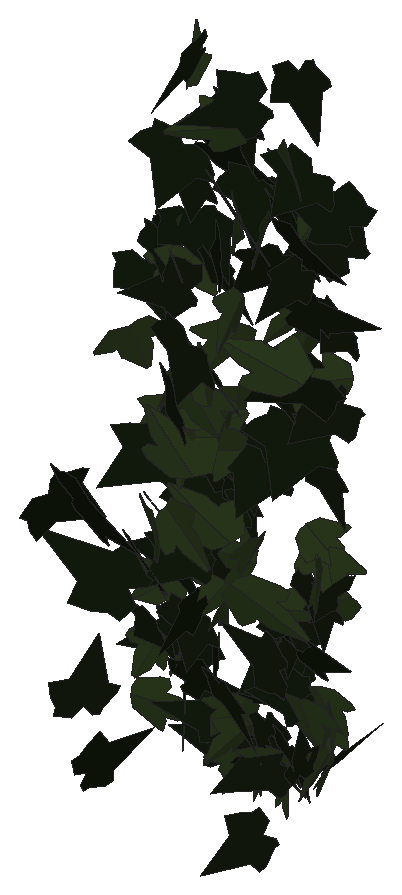
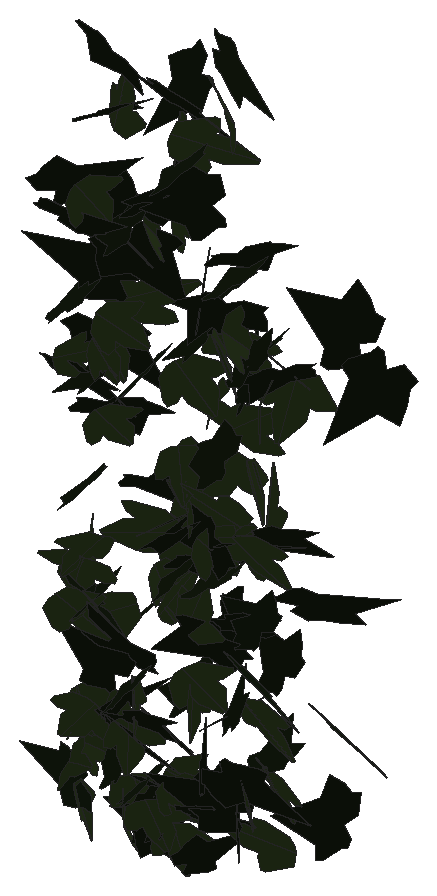
# SketchUp Ruby script. Lengths in inches.
U = 1.inch
M = Sketchup.active_model
def pt(a) = Geom::Point3d.new(a.map { |v| v * U })
def face(e, loops, mat)
  f = e.add_face(loops[0].map { |a| pt(a) })
  loops[1..].each { |l| e.add_face(l.map { |a| pt(a) }).erase! }
  f.material = f.back_material = mat if mat
  f
end
# faces: each face lists its corners as indices into pts; further lists are holes
def faces(e, pts, list, mat = nil) = list.each { |f| face(e, (f[0].is_a?(Array) ? f : [f]).map { |l| l.map { |i| pts[i] } }, mat) }
# xy, xz, yz: faces in a plane at the given z, y or x. An outline is a flat list of corners, or four numbers for a rectangle; further outlines are holes
def ring(l) = l.size == 4 ? [[l[0], l[1]], [l[2], l[1]], [l[2], l[3]], [l[0], l[3]]] : l.each_slice(2).to_a
def flat(e, list, mat, &to3) = list.each { |f| face(e, (f[0].is_a?(Array) ? f : [f]).map { |l| ring(l).map { |u, v| to3.(u, v) } }, mat) }
def xy(e, z, list, mat = nil) = flat(e, list, mat) { |x, y| [x, y, z] }
def xz(e, y, list, mat = nil) = flat(e, list, mat) { |x, z| [x, y, z] }
def yz(e, x, list, mat = nil) = flat(e, list, mat) { |y, z| [x, y, z] }
def lines(e, pts, list) = list.each { |a, b| e.add_line(pt(pts[a]), pt(pts[b])) }
# prism: a flat outline (further loops are holes) pulled along v
def prism(e, loops, v, mat = nil)
  f = face(e, loops, mat); d = Geom::Vector3d.new(v.map { |x| x * U })
  f.pushpull(f.normal.samedirection?(d) ? d.length : -d.length)
end
def box(e, o, s, mat = nil) = prism(e, [[o, [o[0] + s[0], o[1], o[2]], [o[0] + s[0], o[1] + s[1], o[2]], [o[0], o[1] + s[1], o[2]]]], [0, 0, s[2]], mat)
def at(x, y, z, deg = 0) = Geom::Transformation.translation(pt([x, y, z])) * Geom::Transformation.rotation(ORIGIN, Z_AXIS, deg.degrees)
def axes(o, x, y, z) = Geom::Transformation.new([*x, 0, *y, 0, *z, 0, *pt(o).to_a, 1])
def part(name) = M.definitions.add(name)
# library, detail: a bought-in or finely detailed component or shape, given as its bounding box
def library(name, o, s) = part(name).tap { |d| box(d.entities, o, s) }
def detail(e, o, s) = box(e.add_group.entities, o, s)
def put(e, d, t, mat = nil) = e.add_instance(d, t).tap { |i| i.material = mat if mat }
def group(e, t, mat = nil) = e.add_group.tap { |g| g.transformation = t; g.material = mat if mat }.entities
root = M.entities
M.materials.add("1026 AP 7946 SUNNY SIDE UP").color = [254, 231, 186]
M.materials.add("efeu1").color = [18, 25, 13]
M.materials.add("efeu2").color = [43, 57, 29]
c1 = part("ivyleaf_9")
p = [[1.54,2.16,1.25],[1.36,2.04,1.19],[-0.21,0.99,0.68],[-0.71,1.11,0.82],[-0.85,0.86,0.67],[-0.8,0.17,0.21],
  [-0.9,-0.01,0.1],[-0.67,-0.16,-0.02],[-0.08,-0.08,-0.05],[-0.03,-0.6,-0.4],[0.65,-0.88,-0.66],[0.83,-0.6,-0.49],
  [1.29,-0.42,-0.43],[1.8125,-0.07,-0.26],[1.21,0.44,0.15]]
faces(c1.entities,p,[[0,1,2,3,4,5,6,7,8,9,10,11,12,13,14]],"efeu1")
c2 = part("ivyleaf_10")
p = [[0,0.5,-0.03],[-0.0625,2.02,-0.43],[-0.19,2.01,-0.46],[-0.54,1.05,-0.29],[-0.52,0.625,-0.18],[-0.83,0.76,-0.28],
  [-1.16,0.64,-0.33],[-1.15,0.33,-0.24],[-0.77,-0.39,0.02],[-0.3,-0.51,0.16],[0.04,-0.48,0.23],[-0.02,2.01,-0.4375],
  [-0.06,2.01,-0.43],[0.04,-0.49,0.23],[0.67,-0.49,0.14],[1.38,0.36,-0.2],[1.375,0.51,-0.24],[0.81,0.65,-0.19],
  [0.62,0.59,-0.15],[0.6,1.09,-0.28],[0.5,1.23,-0.31]]
faces(c2.entities,p,[[0,1,2,3,4,5,6,7,8,9,10],[11,12,0,13,14,15,16,17,18,19,20]],"efeu2")
put(root,c1,axes([114.62,207.98,273.75],[0.2482,-0.1981,0.34373],[0.28085,-0.28405,-0.26157],[0.54338,0.2373,-0.02181]),"1026 AP 7946 SUNNY SIDE UP")
put(root,c1,axes([114.02,208.15,273.55],[-0.02229,-0.02198,-0.42734],[-0.23875,0.38648,-0.01349],[0.60777,0.15101,-0.02098]),"1026 AP 7946 SUNNY SIDE UP")
put(root,c1,axes([116.61,209.73,268.14],[-0.49831,0.10185,-0.0594],[0.071,-0.04894,-0.3416],[-0.17027,-0.31848,0.0314]),"1026 AP 7946 SUNNY SIDE UP")
put(root,c1,axes([114.91,210.2,275.41],[-0.06712,-0.30626,0.23486],[-0.02015,-0.22987,-0.31951],[0.60163,-0.04187,0.0155]),"1026 AP 7946 SUNNY SIDE UP")
put(root,c1,axes([115.61,210.05,278.29],[0.50276,-0.19479,-0.12293],[-0.18455,0.0338,-0.38421],[0.30709,0.33922,-0.02965]),"1026 AP 7946 SUNNY SIDE UP")
put(root,c2,axes([114.29,210.19,272.0625],[-0.33314,0.25497,0.19565],[0.21856,-0.12904,0.34006],[0.44809,0.2525,-0.02041]),"1026 AP 7946 SUNNY SIDE UP")
put(root,c1,axes([113.23,209.89,269.08],[-0.44459,0.21006,-0.05411],[-0.04291,0.05309,0.36219],[0.33822,0.28286,-0.02517]),"1026 AP 7946 SUNNY SIDE UP")
put(root,c2,axes([115.65,210.34,276.28],[-0.00744,-0.21724,0.27933],[0.17282,-0.25942,-0.2127],[0.51985,0.08313,0.07471]),"1026 AP 7946 SUNNY SIDE UP")
put(root,c1,axes([113.74,210.18,271.05],[-0.41644,-0.23212,-0.14016],[-0.18031,-0.07327,0.36183],[-0.38155,0.28797,-0.01802]),"1026 AP 7946 SUNNY SIDE UP")
put(root,c1,axes([114.44,210.51,274.11],[-0.06511,-0.04806,0.37115],[-0.04374,-0.36139,-0.05504],[0.57026,-0.03321,0.03815]),"1026 AP 7946 SUNNY SIDE UP")
put(root,c1,axes([113.22,210.04,267.89],[0.04851,0.05898,0.37667],[0.39457,0.26605,-0.06453],[-0.42758,0.2522,-0.01681]),"1026 AP 7946 SUNNY SIDE UP")
put(root,c2,axes([114.75,210.3,273.41],[0.47491,0.06702,0.23386],[-0.35843,-0.01444,0.31728],[0.09807,-0.37732,0.02712]),"1026 AP 7946 SUNNY SIDE UP")
put(root,c2,axes([115.82,210.4375,271.53],[-0.30148,0.00089,-0.33899],[0.50697,-0.07563,-0.19419],[-0.10344,-0.37326,0.03626]),"1026 AP 7946 SUNNY SIDE UP")
put(root,c1,axes([114.61,210.74,270.83],[-0.11614,0.01292,-0.32557],[0.28583,-0.26394,-0.05641],[-0.40715,-0.18898,0.05327]),"1026 AP 7946 SUNNY SIDE UP")
put(root,c2,axes([115.58,210.43,277.7],[0.19843,-0.25846,-0.2104],[0.03101,0.22278,-0.2786],[0.51561,0.08607,0.09772]),"1026 AP 7946 SUNNY SIDE UP")
put(root,c1,axes([116.1,210.73,270.28],[-0.02052,-0.33182,0.01504],[0.00434,0.01639,0.34219],[-0.52238,0.01317,0.00225]),"1026 AP 7946 SUNNY SIDE UP")
put(root,c1,axes([115.0625,210.77,269.59],[0.21253,-0.27319,0.10023],[0.05342,-0.09341,-0.31437],[0.45369,0.13897,-0.00994]),"1026 AP 7946 SUNNY SIDE UP")
put(root,c2,axes([114.13,210.79,272.02],[0.23931,-0.02385,0.34986],[0.51535,-0.09094,-0.15836],[0.14563,0.361,-0.01452]),"1026 AP 7946 SUNNY SIDE UP")
put(root,c2,axes([116.14,210.875,275.09],[0.19966,0.1981,0.32347],[-0.33152,-0.23322,0.23892],[0.47868,-0.24416,0.03055]),"1026 AP 7946 SUNNY SIDE UP")
put(root,c2,axes([114.28,210.89,273.34],[0.33771,-0.16744,0.17796],[0.18613,-0.1295,-0.28015],[0.33056,0.24398,-0.02407]),"1026 AP 7946 SUNNY SIDE UP")
put(root,c2,axes([114.94,210.86,272.1],[0.32041,0.10412,0.28335],[-0.43817,-0.03639,0.22715],[0.14506,-0.33989,0.06028]),"1026 AP 7946 SUNNY SIDE UP")
put(root,c2,axes([113.32,210.88,274.8],[-0.26462,-0.30768,-0.14131],[0.11753,0.1134,-0.36046],[0.51535,-0.18385,0.00965]),"1026 AP 7946 SUNNY SIDE UP")
put(root,c2,axes([114.85,211.29,273.19],[-0.04701,-0.07544,-0.32505],[-0.29559,-0.25369,0.07946],[-0.41494,0.18927,-0.01978]),"1026 AP 7946 SUNNY SIDE UP")
put(root,c1,axes([114.26,211.21,279.59],[-0.37275,0.17604,-0.228],[0.2485,-0.15858,-0.30389],[-0.37022,-0.28368,0.02558]),"1026 AP 7946 SUNNY SIDE UP")
put(root,c1,axes([113.14,211.35,270.75],[0.06292,-0.16076,0.29588],[0.14529,-0.27316,-0.17184],[0.49803,0.1,0.01275]),"1026 AP 7946 SUNNY SIDE UP")
put(root,c1,axes([116.38,210.9375,268.58],[0.06624,0.0945,0.26304],[-0.05065,0.25775,-0.09149],[-0.42429,-0.01602,0.05199]),"1026 AP 7946 SUNNY SIDE UP")
put(root,c2,axes([114.92,211.35,268.58],[-0.06145,-0.18285,0.24697],[-0.02077,-0.24151,-0.19257],[0.47494,-0.03422,0.02354]),"1026 AP 7946 SUNNY SIDE UP")
put(root,c2,axes([114.54,211,274.17],[-0.04366,0.27735,-0.1678],[-0.04019,0.16266,0.28799],[0.50542,0.03689,0.0084]),"1026 AP 7946 SUNNY SIDE UP")
put(root,c1,axes([113.53,211.37,272.68],[-0.41707,-0.16252,0.1354],[-0.15216,-0.0944,-0.31976],[0.29235,-0.28099,0.02674]),"1026 AP 7946 SUNNY SIDE UP")
put(root,c2,axes([116.4,211.38,268.5625],[0.07382,-0.16814,0.26457],[0.11941,-0.24636,-0.18124],[0.46896,0.0892,0.0045]),"1026 AP 7946 SUNNY SIDE UP")
put(root,c1,axes([116.17,211.43,278.16],[-0.28513,-0.22686,0.14425],[-0.04325,-0.15402,-0.29199],[0.41803,-0.17067,0.06818]),"1026 AP 7946 SUNNY SIDE UP")
put(root,c1,axes([114.06,211.35,271.23],[-0.36398,-0.14775,0.07439],[-0.0783,-0.05738,-0.28243],[0.24706,-0.23586,0.0201]),"1026 AP 7946 SUNNY SIDE UP")
put(root,c2,axes([116,211.21,278.06],[-0.41765,0.22798,0.02135],[0.0447,0.00333,0.35998],[0.357,0.2663,-0.02009]),"1026 AP 7946 SUNNY SIDE UP")
put(root,c1,axes([116.02,211.41,273.83],[-0.37975,-0.25076,-0.02997],[0.05641,0.00378,-0.35785],[0.39266,-0.24306,0.02243]),"1026 AP 7946 SUNNY SIDE UP")
put(root,c1,axes([115.6,211.36,268.26],[-0.48011,-0.00343,0.03807],[-0.05734,-0.02996,-0.31329],[0.01098,-0.3061,0.02843]),"1026 AP 7946 SUNNY SIDE UP")
put(root,c1,axes([116.24,211.31,274.88],[0.11343,0.02058,-0.34173],[-0.39286,-0.22066,-0.07134],[-0.34489,0.25812,-0.03112]),"1026 AP 7946 SUNNY SIDE UP")
put(root,c2,axes([116.26,211.48,271.52],[0.07278,-0.04443,0.33542],[0.3182,-0.25553,-0.067],[0.40761,0.20742,-0.00759]),"1026 AP 7946 SUNNY SIDE UP")
put(root,c1,axes([114.05,211.24,275.6],[-0.39008,0.18656,0.09253],[-0.14389,0.02513,-0.31775],[-0.29125,-0.26228,0.03305]),"1026 AP 7946 SUNNY SIDE UP")
put(root,c1,axes([115.75,211.48,268.51],[0.12541,-0.23672,0.15952],[0.04616,-0.15448,-0.25756],[0.44355,0.08301,-0.01829]),"1026 AP 7946 SUNNY SIDE UP")
put(root,c1,axes([115.96,211.42,276.47],[-0.45666,0.04908,-0.12472],[0.1783,-0.05318,-0.30206],[-0.10281,-0.31023,0.03014]),"1026 AP 7946 SUNNY SIDE UP")
put(root,c1,axes([115.25,211.5,273.01],[-0.3177,-0.20742,-0.00521],[0.02705,-0.01136,-0.29764],[0.32507,-0.20176,0.01968]),"1026 AP 7946 SUNNY SIDE UP")
put(root,c1,axes([114.31,211.53,272.17],[-0.26387,-0.29403,-0.02556],[0.04593,0.00992,-0.34808],[0.46148,-0.16911,0.02003]),"1026 AP 7946 SUNNY SIDE UP")
put(root,c2,axes([114.57,211.54,278.33],[-0.10653,-0.03707,0.34364],[-0.33223,-0.25997,-0.07544],[0.41046,-0.22004,0.02812]),"1026 AP 7946 SUNNY SIDE UP")
put(root,c1,axes([115.76,211.52,276.81],[0.17683,-0.14292,0.29286],[0.2571,-0.23369,-0.18851],[0.43052,0.19826,-0.00771]),"1026 AP 7946 SUNNY SIDE UP")
put(root,c2,axes([115.09,211.56,267.95],[-0.06022,0.08972,-0.28633],[0.07867,-0.27468,-0.09987],[-0.45322,-0.0596,0.02071]),"1026 AP 7946 SUNNY SIDE UP")
put(root,c1,axes([115.86,211.57,269.33],[-0.14624,-0.02373,0.27968],[-0.27618,-0.21428,-0.08249],[0.3279,-0.19106,0.05525]),"1026 AP 7946 SUNNY SIDE UP")
put(root,c2,axes([116.1,211.375,269.36],[-0.4555,0.03515,-0.04957],[0.06964,-0.03423,-0.2994],[-0.06306,-0.29168,0.02741]),"1026 AP 7946 SUNNY SIDE UP")
put(root,c2,axes([114.86,211.58,271.25],[-0.04933,0.19465,0.27143],[0.08984,-0.25624,0.20138],[0.50577,0.0645,-0.0093]),"1026 AP 7946 SUNNY SIDE UP")
put(root,c1,axes([113.87,211.6,269.97],[-0.09179,-0.27319,0.09744],[0.00866,-0.0991,-0.28725],[0.45531,-0.05319,0.02511]),"1026 AP 7946 SUNNY SIDE UP")
put(root,c1,axes([113.18,211.63,269.51],[-0.21964,-0.09653,0.24476],[0.02359,-0.27365,-0.10681],[0.40335,-0.03656,0.13953]),"1026 AP 7946 SUNNY SIDE UP")
put(root,c1,axes([113.35,211.6,271.43],[0.11701,-0.19171,0.2225],[0.17016,-0.18948,-0.21172],[0.42239,0.12944,0.02366]),"1026 AP 7946 SUNNY SIDE UP")
put(root,c1,axes([115.07,211.51,278.92],[-0.5162,0.09639,0.0505],[-0.08921,-0.02219,-0.35055],[-0.14429,-0.3311,0.03608]),"1026 AP 7946 SUNNY SIDE UP")
put(root,c2,axes([115.5,211.49,268.29],[-0.32768,-0.17493,0.08808],[-0.08486,-0.06994,-0.2801],[0.29489,-0.21451,0.01727]),"1026 AP 7946 SUNNY SIDE UP")
put(root,c2,axes([115.15,211.63,276.87],[0.18633,-0.17931,0.23549],[0.18012,-0.19923,-0.22236],[0.42119,0.16452,-0.00909]),"1026 AP 7946 SUNNY SIDE UP")
put(root,c1,axes([115.875,211.45,275.78],[0.18203,-0.00969,0.3262],[0.45421,-0.1353,-0.11384],[0.20469,0.30885,-0.03748]),"1026 AP 7946 SUNNY SIDE UP")
put(root,c1,axes([115.54,211.54,276.51],[0.06927,0.17335,-0.28918],[-0.12559,-0.27019,-0.18574],[-0.50468,0.09103,0.00653]),"1026 AP 7946 SUNNY SIDE UP")
put(root,c2,axes([115.04,211.54,271.62],[0.00025,-0.29987,0.04476],[0.00009,-0.04515,-0.30919],[0.47683,0.00017,0.00003]),"1026 AP 7946 SUNNY SIDE UP")
put(root,c2,axes([115.5,211.6875,267.8],[0.12953,-0.05535,0.29042],[0.30217,-0.20783,-0.10099],[0.33646,0.20796,-0.02111]),"1026 AP 7946 SUNNY SIDE UP")
put(root,c2,axes([114.57,211.65,274.89],[-0.23102,-0.26351,0.17505],[-0.05216,-0.17516,-0.30771],[0.49153,-0.14244,0.04962]),"1026 AP 7946 SUNNY SIDE UP")
put(root,c1,axes([115.22,211.55,274.71],[0.22419,-0.283,-0.09671],[-0.0821,0.07694,-0.32579],[0.46079,0.1514,-0.011]),"1026 AP 7946 SUNNY SIDE UP")
put(root,c2,axes([113.98,211.51,273.71],[-0.48706,-0.06532,-0.13138],[0.20862,-0.01839,-0.32333],[0.08368,-0.33433,0.04142]),"1026 AP 7946 SUNNY SIDE UP")
put(root,c1,axes([114.24,211.76,275.89],[-0.02599,0.04091,0.33293],[-0.09965,-0.31757,0.03625],[0.50206,-0.06092,0.02443]),"1026 AP 7946 SUNNY SIDE UP")
put(root,c2,axes([116.34,211.6875,269.23],[-0.06933,0.17317,-0.20936],[0.06867,-0.19953,-0.1852],[-0.41537,-0.06189,0.00433]),"1026 AP 7946 SUNNY SIDE UP")
put(root,c2,axes([113.12,211.62,269.32],[0.40185,-0.18584,-0.02249],[-0.04965,-0.00821,-0.32455],[0.28982,0.25628,-0.02442]),"1026 AP 7946 SUNNY SIDE UP")
put(root,c1,axes([116.5,211.7,274.35],[-0.52552,-0.00842,-0.0104],[0.01703,-0.03295,-0.34291],[0.01162,-0.33274,0.03225]),"1026 AP 7946 SUNNY SIDE UP")
put(root,c2,axes([113.48,211.57,273.72],[0.12337,-0.28271,-0.08316],[-0.03456,0.076,-0.30181],[0.46032,0.08148,-0.00037]),"1026 AP 7946 SUNNY SIDE UP")
put(root,c1,axes([113.58,211.77,268.53],[-0.05298,-0.01654,-0.30284],[0.40257,-0.14758,-0.02255],[-0.22834,-0.25636,0.03051]),"1026 AP 7946 SUNNY SIDE UP")
put(root,c1,axes([112.97,211.65,275.47],[-0.0378,-0.28014,-0.13285],[0.05584,0.12437,-0.288],[0.48065,-0.03648,0.02301]),"1026 AP 7946 SUNNY SIDE UP")
put(root,c1,axes([115.99,211.83,271.06],[0.0335,-0.29784,0.15273],[0.0072,-0.14998,-0.30844],[0.52428,0.02109,-0.00552]),"1026 AP 7946 SUNNY SIDE UP")
put(root,c2,axes([115.74,211.43,270.85],[-0.04182,-0.06601,-0.29638],[0.30756,0.21189,-0.06756],[0.34683,-0.19586,0.02418]),"1026 AP 7946 SUNNY SIDE UP")
put(root,c1,axes([115.73,211.73,270.04],[0.10462,-0.08213,0.29047],[0.28629,-0.21591,-0.11013],[0.36322,0.19384,0.00314]),"1026 AP 7946 SUNNY SIDE UP")
put(root,c2,axes([113,211.64,268.32],[0.01434,-0.02948,-0.32352],[0.48721,-0.05705,0.01446],[-0.09138,-0.30878,0.02633]),"1026 AP 7946 SUNNY SIDE UP")
put(root,c2,axes([114.68,211.68,267.92],[-0.27109,-0.19139,0.0564],[-0.03384,-0.05552,-0.26483],[0.31165,-0.17251,0.02031]),"1026 AP 7946 SUNNY SIDE UP")
put(root,c2,axes([113.66,211.71,275.7],[0.4504,0.05989,-0.14816],[-0.21241,-0.05588,-0.30076],[-0.12302,0.31576,-0.02315]),"1026 AP 7946 SUNNY SIDE UP")
put(root,c1,axes([114.9,211.8,277.4],[-0.16549,-0.29489,-0.01607],[0.01458,0.01147,-0.32245],[0.46397,-0.10554,0.0044]),"1026 AP 7946 SUNNY SIDE UP")
put(root,c1,axes([114.34,211.72,268.36],[-0.25704,0.06606,0.20435],[-0.32788,-0.04079,-0.16359],[-0.01423,-0.25349,0.07795]),"1026 AP 7946 SUNNY SIDE UP")
put(root,c2,axes([114.58,211.77,268.69],[-0.21309,-0.19735,0.15338],[-0.08056,-0.14497,-0.24502],[0.38137,-0.1409,0.03395]),"1026 AP 7946 SUNNY SIDE UP")
put(root,c1,axes([114.89,211.79,268.15],[0.24192,-0.19898,0.18962],[0.16936,-0.15076,-0.25993],[0.39243,0.18772,-0.00472]),"1026 AP 7946 SUNNY SIDE UP")
put(root,c1,axes([116.51,211.57,271.24],[-0.26812,0.25713,0.06017],[-0.08185,0.0336,-0.31665],[-0.40594,-0.17661,0.02411]),"1026 AP 7946 SUNNY SIDE UP")
put(root,c1,axes([114.99,211.74,268.03],[-0.06458,0.15674,-0.21547],[0.06648,-0.20586,-0.16798],[-0.40669,-0.05854,0.00676]),"1026 AP 7946 SUNNY SIDE UP")
put(root,c1,axes([115.14,211.73,268.59],[0.18615,-0.26162,-0.0448],[-0.02637,0.03852,-0.2956],[0.4158,0.11957,0.00131]),"1026 AP 7946 SUNNY SIDE UP")
put(root,c2,axes([116.33,211.9,274.63],[-0.06983,0.04405,0.30587],[-0.05695,-0.29848,0.03832],[0.46812,-0.02974,0.05029]),"1026 AP 7946 SUNNY SIDE UP")
put(root,c1,axes([113.13,211.89,275.76],[0.01647,-0.28515,0.11083],[0.00017,-0.10926,-0.29457],[0.48012,0.00982,-0.0037]),"1026 AP 7946 SUNNY SIDE UP")
put(root,c1,axes([115.64,211.84,279.44],[-0.21032,-0.1066,-0.29479],[0.47384,0.00052,-0.14562],[0.07188,-0.31532,0.09736]),"1026 AP 7946 SUNNY SIDE UP")
put(root,c1,axes([113.65,211.9,272.7],[-0.33419,-0.02522,0.19326],[-0.23595,-0.14979,-0.19661],[0.18178,-0.24079,0.1001]),"1026 AP 7946 SUNNY SIDE UP")
put(root,c2,axes([114.41,211.6875,271.23],[-0.43068,0.15889,-0.07601],[-0.07964,0.061,0.32541],[0.26432,0.27727,-0.0258]),"1026 AP 7946 SUNNY SIDE UP")
put(root,c1,axes([115.62,211.64,270.3125],[-0.33927,0.13586,0.177],[0.23525,-0.08325,0.26207],[0.25026,0.26245,-0.0064]),"1026 AP 7946 SUNNY SIDE UP")
put(root,c1,axes([113.96,211.7,271.14],[-0.00956,-0.08492,-0.28627],[0.32455,0.19371,-0.06462],[0.32056,-0.19865,0.05688]),"1026 AP 7946 SUNNY SIDE UP")
put(root,c2,axes([114.22,211.92,270.54],[-0.23378,-0.19982,0.19993],[-0.05444,-0.20624,-0.24587],[0.43585,-0.13294,0.07652]),"1026 AP 7946 SUNNY SIDE UP")
put(root,c2,axes([115.69,211.85,275.05],[-0.07072,-0.27578,0.09656],[0.01608,-0.09786,-0.28733],[0.45852,-0.03911,0.02497]),"1026 AP 7946 SUNNY SIDE UP")
put(root,c2,axes([113.3,211.75,270.31],[0.36191,-0.1317,-0.18318],[-0.26035,0.06607,-0.27197],[0.22939,0.28277,-0.01966]),"1026 AP 7946 SUNNY SIDE UP")
put(root,c1,axes([114.06,211.9,269.03],[-0.01933,0.10876,0.26695],[-0.0981,-0.25333,0.10526],[0.42994,-0.05291,0.03602]),"1026 AP 7946 SUNNY SIDE UP")
put(root,c1,axes([116.26,212.02,275.44],[-0.13567,-0.17192,0.24799],[-0.01643,-0.2498,-0.18835],[0.46608,-0.05884,0.06555]),"1026 AP 7946 SUNNY SIDE UP")
put(root,c2,axes([113.86,211.61,278.92],[0.31926,-0.18133,0.26626],[-0.2622,0.20077,0.28013],[-0.42311,-0.26125,0.02731]),"1026 AP 7946 SUNNY SIDE UP")
put(root,c2,axes([115.68,211.95,273.95],[-0.2174,-0.17602,0.19137],[-0.01042,-0.20962,-0.20981],[0.40341,-0.10027,0.09771]),"1026 AP 7946 SUNNY SIDE UP")
put(root,c2,axes([115.57,211.98,275.46],[-0.09651,-0.19956,0.24018],[-0.07025,-0.23058,-0.21575],[0.47878,-0.07406,0.01676]),"1026 AP 7946 SUNNY SIDE UP")
put(root,c2,axes([116.09,211.8,269.36],[-0.38423,0.02888,-0.12019],[0.17468,-0.04755,-0.25176],[-0.07277,-0.26664,0.03025]),"1026 AP 7946 SUNNY SIDE UP")
put(root,c2,axes([113.91,211.99,272.67],[-0.06553,-0.23276,0.22396],[0.01644,-0.22145,-0.24202],[0.50195,-0.02313,0.03716]),"1026 AP 7946 SUNNY SIDE UP")
put(root,c2,axes([113.82,211.71,272.99],[0.33062,0.01429,-0.27454],[0.40931,0.06426,0.21545],[0.09306,-0.33338,0.02773]),"1026 AP 7946 SUNNY SIDE UP")
put(root,c1,axes([114.2,211.98,267.82],[-0.07617,0.00683,0.28909],[-0.3549,-0.17018,-0.03687],[0.2623,-0.22827,0.03406]),"1026 AP 7946 SUNNY SIDE UP")
put(root,c1,axes([115.69,211.83,269.34],[-0.37947,0.11767,0.09346],[-0.14007,0.02231,-0.27585],[-0.18619,-0.25662,0.01704]),"1026 AP 7946 SUNNY SIDE UP")
put(root,c1,axes([115.28,211.98,269.63],[-0.36981,-0.12254,0.04337],[-0.04481,-0.03766,-0.27265],[0.19911,-0.23606,0.01919]),"1026 AP 7946 SUNNY SIDE UP")
put(root,c1,axes([113.64,211.83,268.72],[0.21054,-0.03248,0.28533],[0.39571,-0.11876,-0.14028],[0.18958,0.28397,-0.02406]),"1026 AP 7946 SUNNY SIDE UP")
put(root,c1,axes([116.4,211.97,277.17],[-0.04866,0.04832,0.34079],[-0.4998,-0.10632,-0.01527],[0.16149,-0.31448,0.05543]),"1026 AP 7946 SUNNY SIDE UP")
put(root,c1,axes([114.02,211.83,277.7],[0.42745,-0.07822,0.17101],[0.23445,-0.08014,-0.29015],[0.16928,0.30851,-0.02996]),"1026 AP 7946 SUNNY SIDE UP")
put(root,c2,axes([116.3,211.95,270.95],[-0.23347,-0.11718,0.21765],[-0.22923,-0.15526,-0.19456],[0.30407,-0.20702,0.02044]),"1026 AP 7946 SUNNY SIDE UP")
put(root,c1,axes([113.3,212.06,277.33],[-0.26024,-0.28835,0.04591],[-0.01081,-0.04925,-0.34227],[0.45906,-0.16462,0.01797]),"1026 AP 7946 SUNNY SIDE UP")
put(root,c1,axes([113.84,212.07,272.12],[-0.09155,-0.23129,0.15307],[0.0624,-0.15864,-0.23722],[0.42886,-0.02629,0.06719]),"1026 AP 7946 SUNNY SIDE UP")
put(root,c1,axes([113.65,212,274.06],[0.25591,-0.24689,0.13905],[0.09369,-0.1238,-0.30487],[0.43348,0.17251,-0.01619]),"1026 AP 7946 SUNNY SIDE UP")
put(root,c2,axes([113.43,211.86,269.21],[0.1882,-0.25212,-0.05521],[-0.02155,0.0512,-0.28705],[0.40426,0.1201,0.0104]),"1026 AP 7946 SUNNY SIDE UP")
put(root,c1,axes([113.46,211.76,270.85],[-0.24786,0.22081,0.12416],[-0.13923,0.08285,-0.2781],[-0.36924,-0.17946,0.02152]),"1026 AP 7946 SUNNY SIDE UP")
put(root,c1,axes([114.01,211.91,275.8],[0.25772,-0.25706,-0.0366],[-0.03982,0.02424,-0.31381],[0.40579,0.16564,-0.00756]),"1026 AP 7946 SUNNY SIDE UP")
put(root,c2,axes([116.09,211.88,271.6],[0.43199,0.10045,0.07164],[0.11376,0.00241,-0.30048],[-0.15416,0.28325,-0.02098]),"1026 AP 7946 SUNNY SIDE UP")
put(root,c2,axes([115.28,211.79,269.96],[0.11575,-0.2512,-0.14176],[0.00399,0.14119,-0.26608],[0.44927,0.06347,0.03888]),"1026 AP 7946 SUNNY SIDE UP")
put(root,c1,axes([113.44,212.07,270.25],[-0.09284,-0.0287,0.28995],[-0.04442,-0.28564,-0.03776],[0.44288,-0.03467,0.05699]),"1026 AP 7946 SUNNY SIDE UP")
put(root,c1,axes([114.4,212.03,272.03],[0.10543,-0.26447,0.07585],[0.00333,-0.07684,-0.28103],[0.4323,0.06509,-0.01633]),"1026 AP 7946 SUNNY SIDE UP")
put(root,c1,axes([113.1,212.12,275.68],[0.02833,-0.20987,0.25527],[0.06398,-0.24596,-0.21805],[0.50801,0.04268,0.01322]),"1026 AP 7946 SUNNY SIDE UP")
put(root,c2,axes([114.44,211.89,273.76],[-0.21898,-0.26539,-0.01082],[0.01812,0.00411,-0.30862],[0.41715,-0.1395,0.00773]),"1026 AP 7946 SUNNY SIDE UP")
put(root,c1,axes([115.74,211.92,274.6875],[0.26728,-0.23501,-0.04753],[-0.01495,0.04829,-0.29778],[0.37589,0.16903,0.02196]),"1026 AP 7946 SUNNY SIDE UP")
put(root,c1,axes([113.82,211.99,272.84],[-0.02956,-0.04991,-0.3273],[0.50198,0.03323,-0.02466],[0.05741,-0.31624,0.04715]),"1026 AP 7946 SUNNY SIDE UP")
put(root,c1,axes([115.2,212.02,277.02],[0.22446,-0.26932,0.07575],[0.04024,-0.07134,-0.31424],[0.43777,0.14465,-0.00995]),"1026 AP 7946 SUNNY SIDE UP")
put(root,c2,axes([114.26,211.82,270.23],[0.04048,-0.25039,-0.14764],[0.01584,0.14315,-0.25752],[0.45226,0.0174,0.02223]),"1026 AP 7946 SUNNY SIDE UP")
put(root,c1,axes([113.68,211.91,276.34],[-0.15779,-0.21161,-0.23146],[0.16119,0.19865,-0.24004],[0.4563,-0.14335,0.00476]),"1026 AP 7946 SUNNY SIDE UP")
put(root,c2,axes([116.09,211.93,268.14],[0.11059,-0.26758,-0.02727],[-0.01281,0.02366,-0.28488],[0.42238,0.07078,-0.0015]),"1026 AP 7946 SUNNY SIDE UP")
put(root,c1,axes([115.18,212.125,270.08],[0.01841,-0.26326,0.14825],[-0.01082,-0.1457,-0.27207],[0.47277,0.00692,-0.012]),"1026 AP 7946 SUNNY SIDE UP")
put(root,c1,axes([114.4,212.04,272.72],[-0.03083,-0.29481,-0.03651],[0.02215,0.03287,-0.30395],[0.46606,-0.02106,0.01203]),"1026 AP 7946 SUNNY SIDE UP")
put(root,c2,axes([114.31,211.88,273.35],[0.11831,-0.27378,-0.09556],[0.0242,0.09793,-0.28918],[0.45311,0.06626,0.0404]),"1026 AP 7946 SUNNY SIDE UP")
put(root,c2,axes([115.88,212.1,277.32],[-0.1378,-0.24582,0.20741],[0.037,-0.21468,-0.25894],[0.49965,-0.0519,0.07638]),"1026 AP 7946 SUNNY SIDE UP")
put(root,c2,axes([115.67,212.05,275.05],[-0.02105,-0.26331,0.13226],[0.04292,-0.13057,-0.27056],[0.45965,0.00013,0.03132]),"1026 AP 7946 SUNNY SIDE UP")
put(root,c2,axes([115.28,211.92,269.4],[-0.20749,-0.25299,-0.03958],[0.04344,0.02727,-0.29354],[0.39968,-0.1343,0.01136]),"1026 AP 7946 SUNNY SIDE UP")
put(root,c2,axes([114.88,211.99,268.35],[-0.31999,-0.13895,0.09503],[-0.08907,-0.0806,-0.25213],[0.2474,-0.20874,0.03214]),"1026 AP 7946 SUNNY SIDE UP")
put(root,c1,axes([113.55,212.04,269.38],[-0.00739,-0.04492,-0.32203],[-0.35064,-0.22054,0.03484],[-0.35105,0.22122,-0.02802]),"1026 AP 7946 SUNNY SIDE UP")
put(root,c1,axes([115.9,212.07,272.91],[0.11491,-0.27628,0.03144],[0.0022,-0.03281,-0.29452],[0.43735,0.07276,-0.00678]),"1026 AP 7946 SUNNY SIDE UP")
put(root,c2,axes([115.93,211.84,271.95],[0.14064,0.24808,0.14712],[0.10079,0.12695,-0.27048],[-0.43754,0.10898,-0.01502]),"1026 AP 7946 SUNNY SIDE UP")
put(root,c2,axes([113.35,212.17,276.1],[0.13369,-0.21275,0.25527],[0.12157,-0.23694,-0.23715],[0.50042,0.1144,-0.01058]),"1026 AP 7946 SUNNY SIDE UP")
put(root,c1,axes([114.25,212.14,278.23],[0.06561,-0.29637,0.10351],[0.03105,-0.10037,-0.30887],[0.49194,0.04586,0.00569]),"1026 AP 7946 SUNNY SIDE UP")
put(root,c2,axes([113.7,211.99,275.73],[0.23155,-0.27113,-0.02762],[-0.03198,0.0177,-0.3176],[0.42698,0.14836,-0.00881]),"1026 AP 7946 SUNNY SIDE UP")
put(root,c1,axes([116.41,211.9,276.71],[-0.46077,-0.07923,-0.13463],[-0.21085,-0.00024,0.31099],[-0.11401,0.32067,-0.03104]),"1026 AP 7946 SUNNY SIDE UP")
put(root,c1,axes([113.34,212.1875,276.89],[-0.05229,-0.2689,0.15441],[0.05096,-0.15449,-0.27622],[0.48255,-0.01282,0.0459]),"1026 AP 7946 SUNNY SIDE UP")
put(root,c1,axes([116.23,211.8,268.26],[-0.0392,0.30375,-0.0231],[-0.00251,0.0241,0.31411],[0.47911,0.02498,-0.00024]),"1026 AP 7946 SUNNY SIDE UP")
put(root,c1,axes([114.48,212.17,272.89],[-0.12083,-0.25562,0.10389],[0.02194,-0.10969,-0.27221],[0.43238,-0.06587,0.04284]),"1026 AP 7946 SUNNY SIDE UP")
put(root,c2,axes([113.17,211.76,274.9],[-0.06668,0.17314,-0.27732],[-0.07043,0.26667,0.18485],[0.49964,0.06069,-0.01095]),"1026 AP 7946 SUNNY SIDE UP")
put(root,c2,axes([116.08,212.13,268.74],[0.03429,0.16625,-0.24488],[-0.0613,-0.23549,-0.17405],[-0.45321,0.04443,0.00501]),"1026 AP 7946 SUNNY SIDE UP")
put(root,c2,axes([113.24,212.03,272.92],[0.40747,-0.02498,-0.1783],[-0.27418,-0.01706,-0.26673],[0.01768,0.31108,-0.02711]),"1026 AP 7946 SUNNY SIDE UP")
